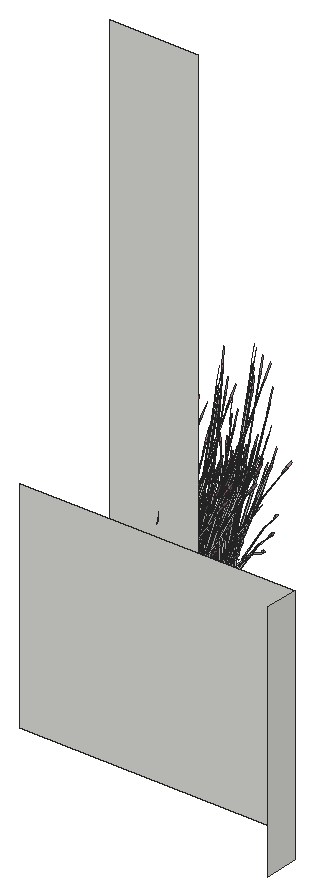
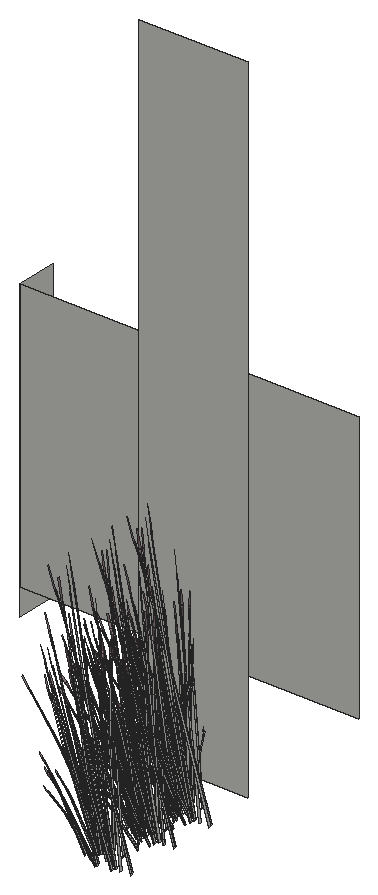
# SketchUp Ruby script. Lengths in inches.
U = 1.inch
M = Sketchup.active_model
def pt(a) = Geom::Point3d.new(a.map { |v| v * U })
def face(e, loops, mat)
  f = e.add_face(loops[0].map { |a| pt(a) })
  loops[1..].each { |l| e.add_face(l.map { |a| pt(a) }).erase! }
  f.material = f.back_material = mat if mat
  f
end
# faces: each face lists its corners as indices into pts; further lists are holes
def faces(e, pts, list, mat = nil) = list.each { |f| face(e, (f[0].is_a?(Array) ? f : [f]).map { |l| l.map { |i| pts[i] } }, mat) }
# xy, xz, yz: faces in a plane at the given z, y or x. An outline is a flat list of corners, or four numbers for a rectangle; further outlines are holes
def ring(l) = l.size == 4 ? [[l[0], l[1]], [l[2], l[1]], [l[2], l[3]], [l[0], l[3]]] : l.each_slice(2).to_a
def flat(e, list, mat, &to3) = list.each { |f| face(e, (f[0].is_a?(Array) ? f : [f]).map { |l| ring(l).map { |u, v| to3.(u, v) } }, mat) }
def xy(e, z, list, mat = nil) = flat(e, list, mat) { |x, y| [x, y, z] }
def xz(e, y, list, mat = nil) = flat(e, list, mat) { |x, z| [x, y, z] }
def yz(e, x, list, mat = nil) = flat(e, list, mat) { |y, z| [x, y, z] }
def lines(e, pts, list) = list.each { |a, b| e.add_line(pt(pts[a]), pt(pts[b])) }
# prism: a flat outline (further loops are holes) pulled along v
def prism(e, loops, v, mat = nil)
  f = face(e, loops, mat); d = Geom::Vector3d.new(v.map { |x| x * U })
  f.pushpull(f.normal.samedirection?(d) ? d.length : -d.length)
end
def box(e, o, s, mat = nil) = prism(e, [[o, [o[0] + s[0], o[1], o[2]], [o[0] + s[0], o[1] + s[1], o[2]], [o[0], o[1] + s[1], o[2]]]], [0, 0, s[2]], mat)
def at(x, y, z, deg = 0) = Geom::Transformation.translation(pt([x, y, z])) * Geom::Transformation.rotation(ORIGIN, Z_AXIS, deg.degrees)
def axes(o, x, y, z) = Geom::Transformation.new([*x, 0, *y, 0, *z, 0, *pt(o).to_a, 1])
def part(name) = M.definitions.add(name)
# library, detail: a bought-in or finely detailed component or shape, given as its bounding box
def library(name, o, s) = part(name).tap { |d| box(d.entities, o, s) }
def detail(e, o, s) = box(e.add_group.entities, o, s)
def put(e, d, t, mat = nil) = e.add_instance(d, t).tap { |i| i.material = mat if mat }
def group(e, t, mat = nil) = e.add_group.tap { |g| g.transformation = t; g.material = mat if mat }.entities
root = M.entities
M.materials.add("LightPink_Translucent").color = [144, 107, 117]
M.materials["LightPink_Translucent"].alpha = 0.75
c1 = part("blade")
p = [[2.15,0.21,22],[0,0.17,0],[0.09,0.45,0],[2.18,0.31,22],[2.29,0.31,22],[0.38,0.45,0],
  [2.48,0.24,33],[2.49,0.24,33],[2.48,0.22,33]]
faces(c1.entities,p,[[0,1,2,3],[4,5,2,3],[6,3,4,7],[8,0,3,6]])
c2 = part("seeds")
p = [[0.3,-0.1,1.38],[-0.01,-0.03,1.59],[-0.01,-0.03,0.03],[0.14,-0.07,-0.07],[0.29,-0.03,3],[0.15,0.01,3.11]]
faces(c2.entities,p,[[0,1,2,3],[1,0,4,5]],"LightPink_Translucent")
c3 = part("blade with seeds")
put(c3.entities,c1,at(0,0,0))
put(c3.entities,c2,axes([2.4,0.25,30.99],[1.5799,-0.05474,1.17369],[-0.12525,1.92788,0.29478],[-0.07173,-0.02425,1.56792]))
xz(root,9,[[351,0,426,60]])
xz(root,51,[[342,6,366,151.99]])
yz(root,426,[[0,-6,9,60]])
put(root,c3,axes([347.36,59.61,7.02],[0.73517,0.0304,0.0643],[-0.02016,0.45906,0.50621],[0.07693,-0.17585,0.77189]))
put(root,c3,axes([347.36,69.44,7.02],[0.73517,0.0304,0.0643],[-0.02016,0.45906,0.50621],[0.07693,-0.17585,0.77189]))
put(root,c3,axes([347.36,81.44,7.02],[0.73517,0.0304,0.0643],[-0.02016,0.45906,0.50621],[0.07693,-0.17585,0.77189]))
put(root,c3,axes([347.27,63.85,5.06],[-0.5037,-0.18761,1.1486],[0.6504,-0.19062,0.84392],[0.17543,0.16147,0.25299]))
put(root,c3,axes([347.27,73.68,5.06],[-0.5037,-0.18761,1.1486],[0.6504,-0.19062,0.84392],[0.17543,0.16147,0.25299]))
put(root,c3,axes([345.48,63.65,4.88],[0.01579,-0.21629,1.43002],[0.75442,-0.24159,-0.30754],[0.23289,0.25887,0.61141]))
put(root,c3,axes([345.48,73.48,4.88],[0.01579,-0.21629,1.43002],[0.75442,-0.24159,-0.30754],[0.23289,0.25887,0.61141]))
put(root,c3,axes([348.09,58.86,7.01],[-0.00864,-0.12985,1.74944],[-0.72937,-0.3753,-0.27667],[0.11277,-0.2275,0.14031]))
put(root,c3,axes([348.09,68.68,7.01],[-0.00864,-0.12985,1.74944],[-0.72937,-0.3753,-0.27667],[0.11277,-0.2275,0.14031]))
put(root,c3,axes([348.09,80.68,7.01],[-0.00864,-0.12985,1.74944],[-0.72937,-0.3753,-0.27667],[0.11277,-0.2275,0.14031]))
put(root,c3,axes([344.57,60.59,4.35],[0.60257,-0.49041,-0.62353],[0.74854,0.44469,-0.16365],[0.24146,-0.12234,1.37633]))
put(root,c3,axes([344.57,70.41,4.35],[0.60257,-0.49041,-0.62353],[0.74854,0.44469,-0.16365],[0.24146,-0.12234,1.37633]))
put(root,c3,axes([344.57,82.41,4.35],[0.60257,-0.49041,-0.62353],[0.74854,0.44469,-0.16365],[0.24146,-0.12234,1.37633]))
put(root,c3,axes([347.12,59.57,7.03],[0.63704,0.44518,0.48003],[-0.67652,0.38394,0.3958],[0.11751,-0.20886,0.9933]))
put(root,c3,axes([347.12,69.4,7.03],[0.63704,0.44518,0.48003],[-0.67652,0.38394,0.3958],[0.11751,-0.20886,0.9933]))
put(root,c3,axes([347.12,81.4,7.03],[0.63704,0.44518,0.48003],[-0.67652,0.38394,0.3958],[0.11751,-0.20886,0.9933]))
put(root,c3,axes([347.22,60.15,4.32],[0.21015,0.56852,-0.30978],[-0.83462,0.16144,0.30978],[0.16826,0.06556,1.38974]))
put(root,c3,axes([347.22,69.98,4.32],[0.21015,0.56852,-0.30978],[-0.83462,0.16144,0.30978],[0.16826,0.06556,1.38974]))
put(root,c3,axes([347.22,81.98,4.32],[0.21015,0.56852,-0.30978],[-0.83462,0.16144,0.30978],[0.16826,0.06556,1.38974]))
put(root,c3,axes([348.79,62.01,4.67],[1.11865,0,0],[0,0.72922,-0.51607],[0,0.16609,1.63711]))
put(root,c3,axes([348.79,71.83,4.67],[1.11865,0,0],[0,0.72922,-0.51607],[0,0.16609,1.63711]))
put(root,c3,axes([345.17,61.06,4.96],[0.90324,-0.43318,-0.29095],[0.60064,0.61207,-0.50002],[0.22285,0.06216,1.59708]))
put(root,c3,axes([345.17,70.89,4.96],[0.90324,-0.43318,-0.29095],[0.60064,0.61207,-0.50002],[0.22285,0.06216,1.59708]))
put(root,c3,axes([345.17,82.89,4.96],[0.90324,-0.43318,-0.29095],[0.60064,0.61207,-0.50002],[0.22285,0.06216,1.59708]))
put(root,c3,axes([347.35,64.71,4.96],[-0.57368,-0.02046,1.0506],[0.37886,-0.43461,0.58006],[0.22663,0.15441,0.8241]))
put(root,c3,axes([347.35,74.53,4.96],[-0.57368,-0.02046,1.0506],[0.37886,-0.43461,0.58006],[0.22663,0.15441,0.8241]))
put(root,c3,axes([347.86,60.99,7.34],[-0.77872,0.09325,0.35414],[-0.20563,-0.53305,-0.4572],[0.22316,-0.14318,0.87481]))
put(root,c3,axes([347.86,70.8125,7.34],[-0.77872,0.09325,0.35414],[-0.20563,-0.53305,-0.4572],[0.22316,-0.14318,0.87481]))
put(root,c3,axes([347.86,82.8125,7.34],[-0.77872,0.09325,0.35414],[-0.20563,-0.53305,-0.4572],[0.22316,-0.14318,0.87481]))
put(root,c3,axes([345.62,59.49,6.17],[-0.16657,0.22426,1.71376],[-0.69879,-0.4641,0.13857],[0.31524,-0.28926,0.73262]))
put(root,c3,axes([345.62,69.32,6.17],[-0.16657,0.22426,1.71376],[-0.69879,-0.4641,0.13857],[0.31524,-0.28926,0.73262]))
put(root,c3,axes([345.62,81.32,6.17],[-0.16657,0.22426,1.71376],[-0.69879,-0.4641,0.13857],[0.31524,-0.28926,0.73262]))
put(root,c3,axes([345.5,64.39,7.33],[0.53309,-0.55848,-0.1216],[0.77201,0.32175,-0.67495],[0.26836,0.15779,1.02557]))
put(root,c3,axes([345.5,74.22,7.33],[0.53309,-0.55848,-0.1216],[0.77201,0.32175,-0.67495],[0.26836,0.15779,1.02557]))
put(root,c3,axes([342.89,60.67,3.89],[-0.88056,0.26122,1.28929],[-0.28027,-0.74951,0.50096],[0.54072,0.01247,1.46642]))
put(root,c3,axes([342.89,70.5,3.89],[-0.88056,0.26122,1.28929],[-0.28027,-0.74951,0.50096],[0.54072,0.01247,1.46642]))
put(root,c3,axes([342.89,82.5,3.89],[-0.88056,0.26122,1.28929],[-0.28027,-0.74951,0.50096],[0.54072,0.01247,1.46642]))
put(root,c3,axes([348.26,61.03,7.33],[-0.82753,-0.35977,-0.1216],[0.47675,-0.52101,-0.67495],[0.2338,-0.18111,1.02557]))
put(root,c3,axes([348.26,70.86,7.33],[-0.82753,-0.35977,-0.1216],[0.47675,-0.52101,-0.67495],[0.2338,-0.18111,1.02557]))
put(root,c3,axes([348.26,82.86,7.33],[-0.82753,-0.35977,-0.1216],[0.47675,-0.52101,-0.67495],[0.2338,-0.18111,1.02557]))
put(root,c3,axes([346.13,64.11,6.97],[0.88277,-0.1551,-0.51099],[0.15442,0.58737,-0.3958],[0.23711,0.16832,0.97773]))
put(root,c3,axes([346.13,73.9375,6.97],[0.88277,-0.1551,-0.51099],[0.15442,0.58737,-0.3958],[0.23711,0.16832,0.97773]))
put(root,c3,axes([346.94,59.52,4.67],[0.55932,-0.6538,0],[0.93577,0.36461,-0.51607],[0.21313,0.08304,1.63711]))
put(root,c3,axes([346.94,69.34,4.67],[0.55932,-0.6538,0],[0.93577,0.36461,-0.51607],[0.21313,0.08304,1.63711]))
put(root,c3,axes([346.94,81.34,4.67],[0.55932,-0.6538,0],[0.93577,0.36461,-0.51607],[0.21313,0.08304,1.63711]))
put(root,c3,axes([347.88,59.23,3.79],[-0.1339,-0.0514,1.76342],[-0.34394,-0.57425,-0.26939],[0.23202,-0.15583,0.30037]))
put(root,c3,axes([347.88,69.06,3.79],[-0.1339,-0.0514,1.76342],[-0.34394,-0.57425,-0.26939],[0.23202,-0.15583,0.30037]))
put(root,c3,axes([347.88,81.06,3.79],[-0.1339,-0.0514,1.76342],[-0.34394,-0.57425,-0.26939],[0.23202,-0.15583,0.30037]))
put(root,c3,axes([347.14,63.41,7.34],[-0.50902,-0.40851,0.35414],[0.58122,-0.38671,-0.4572],[0.29531,0.05884,0.87481]))
put(root,c3,axes([347.14,73.23,7.34],[-0.50902,-0.40851,0.35414],[0.58122,-0.38671,-0.4572],[0.29531,0.05884,0.87481]))
put(root,c3,axes([347.45,59.91,4.3125],[0.83726,0.32623,-0.49651],[-0.50045,0.58498,0],[0.19069,0.0743,1.57504]))
put(root,c3,axes([347.45,69.74,4.3125],[0.83726,0.32623,-0.49651],[-0.50045,0.58498,0],[0.19069,0.0743,1.57504]))
put(root,c3,axes([347.45,81.74,4.3125],[0.83726,0.32623,-0.49651],[-0.50045,0.58498,0],[0.19069,0.0743,1.57504]))
put(root,c3,axes([347.61,63.78,7.02],[-0.04505,0.49615,0.0643],[-0.68022,-0.0136,0.50621],[0.26056,0.05192,0.77189]))
put(root,c3,axes([347.61,73.6,7.02],[-0.04505,0.49615,0.0643],[-0.68022,-0.0136,0.50621],[0.26056,0.05192,0.77189]))
put(root,c3,axes([347.41,64.55,3.79],[0.06518,-0.0942,1.76342],[0.82057,-0.27742,-0.26939],[0.24877,0.14358,0.30037]))
put(root,c3,axes([347.41,74.375,3.79],[0.06518,-0.0942,1.76342],[0.82057,-0.27742,-0.26939],[0.24877,0.14358,0.30037]))
put(root,c3,axes([347.67,63.62,7.03],[-0.65964,0.42992,0.48003],[-0.5689,-0.45657,0.3958],[0.30948,0.0793,0.9933]))
put(root,c3,axes([347.67,73.45,7.03],[-0.65964,0.42992,0.48003],[-0.5689,-0.45657,0.3958],[0.30948,0.0793,0.9933]))
put(root,c3,axes([347.85,60.61,6.97],[-0.22982,-0.59576,-0.51099],[0.87033,-0.10422,-0.3958],[0.24941,-0.16002,0.97773]))
put(root,c3,axes([347.85,70.44,6.97],[-0.22982,-0.59576,-0.51099],[0.87033,-0.10422,-0.3958],[0.24941,-0.16002,0.97773]))
put(root,c3,axes([347.85,82.44,6.97],[-0.22982,-0.59576,-0.51099],[0.87033,-0.10422,-0.3958],[0.24941,-0.16002,0.97773]))
put(root,c3,axes([349.38,63.68,6.22],[-0.17122,-0.54847,-0.03492],[0.80929,-0.12609,-0.15832],[0.169,0.03477,0.52218]))
put(root,c3,axes([349.38,73.51,6.22],[-0.17122,-0.54847,-0.03492],[0.80929,-0.12609,-0.15832],[0.169,0.03477,0.52218]))
put(root,c3,axes([347.98,62.26,7.34],[-0.74348,-0.18202,0.35414],[0.21685,-0.53102,-0.4572],[0.29933,-0.04869,0.87481]))
put(root,c3,axes([347.98,72.09,7.34],[-0.74348,-0.18202,0.35414],[0.21685,-0.53102,-0.4572],[0.29933,-0.04869,0.87481]))
put(root,c3,axes([347.98,84.09,7.34],[-0.74348,-0.18202,0.35414],[0.21685,-0.53102,-0.4572],[0.29933,-0.04869,0.87481]))
put(root,c3,axes([346.23,61.16,4.35],[0.9306,0.10697,-0.62353],[-0.19638,0.65984,-0.16365],[0.27771,0.07995,1.37633]))
put(root,c3,axes([346.23,70.98,4.35],[0.9306,0.10697,-0.62353],[-0.19638,0.65984,-0.16365],[0.27771,0.07995,1.37633]))
put(root,c3,axes([346.23,82.98,4.35],[0.9306,0.10697,-0.62353],[-0.19638,0.65984,-0.16365],[0.27771,0.07995,1.37633]))
put(root,c3,axes([350.19,61.55,4.55],[-0.55463,-0.41721,-0.06488],[0.60744,-0.38228,-0.29416],[0.17212,-0.02691,0.97024]))
put(root,c3,axes([350.19,71.375,4.55],[-0.55463,-0.41721,-0.06488],[0.60744,-0.38228,-0.29416],[0.17212,-0.02691,0.97024]))
put(root,c3,axes([350.19,83.375,4.55],[-0.55463,-0.41721,-0.06488],[0.60744,-0.38228,-0.29416],[0.17212,-0.02691,0.97024]))
put(root,c3,axes([348.92,59.42,5.06],[-0.29798,0.33213,1.1486],[-0.25612,-0.44624,0.84392],[0.24611,-0.11182,0.25299]))
put(root,c3,axes([348.92,69.25,5.06],[-0.29798,0.33213,1.1486],[-0.25612,-0.44624,0.84392],[0.24611,-0.11182,0.25299]))
put(root,c3,axes([348.92,81.25,5.06],[-0.29798,0.33213,1.1486],[-0.25612,-0.44624,0.84392],[0.24611,-0.11182,0.25299]))
put(root,c3,axes([348.5625,60.9,7.02],[0.61415,0.2744,0.0643],[-0.35756,0.39076,0.50621],[0.1969,-0.12633,0.77189]))
put(root,c3,axes([348.5625,70.73,7.02],[0.61415,0.2744,0.0643],[-0.35756,0.39076,0.50621],[0.1969,-0.12633,0.77189]))
put(root,c3,axes([348.5625,82.73,7.02],[0.61415,0.2744,0.0643],[-0.35756,0.39076,0.50621],[0.1969,-0.12633,0.77189]))
put(root,c3,axes([348.39,60.79,7.03],[0.22187,0.60049,0.48003],[-0.87033,0.10422,0.3958],[0.25651,-0.14123,0.9933]))
put(root,c3,axes([348.39,70.61,7.03],[0.22187,0.60049,0.48003],[-0.87033,0.10422,0.3958],[0.25651,-0.14123,0.9933]))
put(root,c3,axes([348.39,82.61,7.03],[0.22187,0.60049,0.48003],[-0.87033,0.10422,0.3958],[0.25651,-0.14123,0.9933]))
put(root,c3,axes([346.04,62.57,6.17],[-0.3323,-0.11241,1.71376],[0.68769,-0.4716,0.13857],[0.42861,0.21275,0.73262]))
put(root,c3,axes([346.04,72.4,6.17],[-0.3323,-0.11241,1.71376],[0.68769,-0.4716,0.13857],[0.42861,0.21275,0.73262]))
put(root,c3,axes([350.3,60.88,7],[-0.11685,-0.00496,1.77383],[-0.48522,-0.53096,-0.16761],[0.19486,-0.17458,0.31391]))
put(root,c3,axes([350.3,70.71,7],[-0.11685,-0.00496,1.77383],[-0.48522,-0.53096,-0.16761],[0.19486,-0.17458,0.31391]))
put(root,c3,axes([350.3,82.71,7],[-0.11685,-0.00496,1.77383],[-0.48522,-0.53096,-0.16761],[0.19486,-0.17458,0.31391]))
put(root,c3,axes([348.49,60.67,6.82],[0.77872,-0.09325,-0.35414],[0.20563,0.53305,0.4572],[0.22316,-0.14318,0.87481]))
put(root,c3,axes([348.49,70.5,6.82],[0.77872,-0.09325,-0.35414],[0.20563,0.53305,0.4572],[0.22316,-0.14318,0.87481]))
put(root,c3,axes([348.49,82.5,6.82],[0.77872,-0.09325,-0.35414],[0.20563,0.53305,0.4572],[0.22316,-0.14318,0.87481]))
put(root,c3,axes([347.875,60.85,7.27],[0.4673,-0.51481,-0.71045],[0.81887,0.36587,0.08574],[0.27902,-0.18652,1.00501]))
put(root,c3,axes([347.875,70.68,7.27],[0.4673,-0.51481,-0.71045],[0.81887,0.36587,0.08574],[0.27902,-0.18652,1.00501]))
put(root,c3,axes([347.875,82.68,7.27],[0.4673,-0.51481,-0.71045],[0.81887,0.36587,0.08574],[0.27902,-0.18652,1.00501]))
put(root,c3,axes([348.66,62.43,7.02],[0.32857,0.44488,0.0643],[-0.59916,0.21775,0.50621],[0.26412,-0.04296,0.77189]))
put(root,c3,axes([348.66,72.25,7.02],[0.32857,0.44488,0.0643],[-0.59916,0.21775,0.50621],[0.26412,-0.04296,0.77189]))
put(root,c3,axes([348.66,84.25,7.02],[0.32857,0.44488,0.0643],[-0.59916,0.21775,0.50621],[0.26412,-0.04296,0.77189]))
put(root,c3,axes([347.87,63.62,6.82],[0.50902,0.40851,-0.35414],[-0.58122,0.38671,0.4572],[0.29531,0.05884,0.87481]))
put(root,c3,axes([347.87,73.45,6.82],[0.50902,0.40851,-0.35414],[-0.58122,0.38671,0.4572],[0.29531,0.05884,0.87481]))
put(root,c3,axes([347.28,63.67,7.33],[0.0479,-0.66354,-0.1216],[0.90696,0.01814,-0.67495],[0.3493,0.04609,1.02557]))
put(root,c3,axes([347.28,73.49,7.33],[0.0479,-0.66354,-0.1216],[0.90696,0.01814,-0.67495],[0.3493,0.04609,1.02557]))
put(root,c3,axes([348.29,62.4375,7.33],[-0.45012,-0.59081,-0.1216],[0.79888,-0.29033,-0.67495],[0.33665,-0.07795,1.02557]))
put(root,c3,axes([348.29,72.27,7.33],[-0.45012,-0.59081,-0.1216],[0.79888,-0.29033,-0.67495],[0.33665,-0.07795,1.02557]))
put(root,c3,axes([348.29,84.27,7.33],[-0.45012,-0.59081,-0.1216],[0.79888,-0.29033,-0.67495],[0.33665,-0.07795,1.02557]))
put(root,c3,axes([348.59,62.27,7.03],[-0.25275,0.59491,0.48003],[-0.83094,-0.20343,0.3958],[0.32677,-0.03575,0.9933]))
put(root,c3,axes([348.59,72.09,7.03],[-0.25275,0.59491,0.48003],[-0.83094,-0.20343,0.3958],[0.32677,-0.03575,0.9933]))
put(root,c3,axes([348.59,84.09,7.03],[-0.25275,0.59491,0.48003],[-0.83094,-0.20343,0.3958],[0.32677,-0.03575,0.9933]))
put(root,c3,axes([348.07,63.27,7.01],[0.19191,-0.01103,1.74944],[0.52639,-0.5069,-0.27667],[0.34136,0.06691,0.14031]))
put(root,c3,axes([348.07,73.1,7.01],[0.19191,-0.01103,1.74944],[0.52639,-0.5069,-0.27667],[0.34136,0.06691,0.14031]))
put(root,c3,axes([348.26,61.93,6.97],[0.24236,-0.59349,-0.51099],[0.83094,0.20343,-0.3958],[0.33455,-0.05442,0.97773]))
put(root,c3,axes([348.26,71.76,6.97],[0.24236,-0.59349,-0.51099],[0.83094,0.20343,-0.3958],[0.33455,-0.05442,0.97773]))
put(root,c3,axes([348.26,83.76,6.97],[0.24236,-0.59349,-0.51099],[0.83094,0.20343,-0.3958],[0.33455,-0.05442,0.97773]))
put(root,c3,axes([350.34,62.31,5.06],[-0.55274,0.10771,1.1486],[0.26018,-0.44517,0.84392],[0.29323,0.03046,0.25299]))
put(root,c3,axes([350.34,72.14,5.06],[-0.55274,0.10771,1.1486],[0.26018,-0.44517,0.84392],[0.29323,0.03046,0.25299]))
put(root,c3,axes([350.34,84.14,5.06],[-0.55274,0.10771,1.1486],[0.26018,-0.44517,0.84392],[0.29323,0.03046,0.25299]))
put(root,c3,axes([348.55,60.375,4.88],[-0.31959,-0.01933,1.43002],[-0.32741,-0.51843,-0.30754],[0.39262,-0.14666,0.61141]))
put(root,c3,axes([348.55,70.2,4.88],[-0.31959,-0.01933,1.43002],[-0.32741,-0.51843,-0.30754],[0.39262,-0.14666,0.61141]))
put(root,c3,axes([348.55,82.2,4.88],[-0.31959,-0.01933,1.43002],[-0.32741,-0.51843,-0.30754],[0.39262,-0.14666,0.61141]))
put(root,c3,axes([348.76,62.2,6.82],[0.74348,0.18202,-0.35414],[-0.21685,0.53102,0.4572],[0.29933,-0.04869,0.87481]))
put(root,c3,axes([348.76,72.03,6.82],[0.74348,0.18202,-0.35414],[-0.21685,0.53102,0.4572],[0.29933,-0.04869,0.87481]))
put(root,c3,axes([348.76,84.03,6.82],[0.74348,0.18202,-0.35414],[-0.21685,0.53102,0.4572],[0.29933,-0.04869,0.87481]))
put(root,c3,axes([347.33,63.35,7.27],[0.89428,0.01571,-0.71045],[-0.06006,0.66153,0.08574],[0.37886,0.06981,1.00501]))
put(root,c3,axes([347.33,73.17,7.27],[0.89428,0.01571,-0.71045],[-0.06006,0.66153,0.08574],[0.37886,0.06981,1.00501]))
put(root,c3,axes([349.14,62.1,4.28],[-0.57619,0.0783,1.41583],[-0.09171,-0.62326,0.08104],[0.40356,-0.09434,0.80566]))
put(root,c3,axes([349.14,71.93,4.28],[-0.57619,0.0783,1.41583],[-0.09171,-0.62326,0.08104],[0.40356,-0.09434,0.80566]))
put(root,c3,axes([349.14,83.93,4.28],[-0.57619,0.0783,1.41583],[-0.09171,-0.62326,0.08104],[0.40356,-0.09434,0.80566]))
put(root,c3,axes([349.77,61.69,3.79],[-0.04675,-0.09906,1.76342],[0.32428,-0.57943,-0.26939],[0.32711,-0.00833,0.30037]))
put(root,c3,axes([349.77,71.52,3.79],[-0.04675,-0.09906,1.76342],[0.32428,-0.57943,-0.26939],[0.32711,-0.00833,0.30037]))
put(root,c3,axes([349.77,83.52,3.79],[-0.04675,-0.09906,1.76342],[0.32428,-0.57943,-0.26939],[0.32711,-0.00833,0.30037]))
put(root,c3,axes([350.09,64.19,7],[-0.08089,-0.05712,1.77383],[0.17695,-0.61228,-0.16761],[0.31864,-0.03912,0.31391]))
put(root,c3,axes([350.09,74.02,7],[-0.08089,-0.05712,1.77383],[0.17695,-0.61228,-0.16761],[0.31864,-0.03912,0.31391]))
put(root,c3,axes([350.09,86.02,7],[-0.08089,-0.05712,1.77383],[0.17695,-0.61228,-0.16761],[0.31864,-0.03912,0.31391]))
put(root,c3,axes([346.74,61.55,6.17],[-0.37107,0.01478,1.71376],[0.24616,-0.64047,0.13857],[0.5288,0.03961,0.73262]))
put(root,c3,axes([346.74,71.37,6.17],[-0.37107,0.01478,1.71376],[0.24616,-0.64047,0.13857],[0.5288,0.03961,0.73262]))
put(root,c3,axes([346.74,83.37,6.17],[-0.37107,0.01478,1.71376],[0.24616,-0.64047,0.13857],[0.5288,0.03961,0.73262]))
put(root,c3,axes([348.1,62.15,7.27],[0.78611,-0.28816,-0.71045],[0.4381,0.59317,0.08574],[0.37982,-0.06738,1.00501]))
put(root,c3,axes([348.1,71.97,7.27],[0.78611,-0.28816,-0.71045],[0.4381,0.59317,0.08574],[0.37982,-0.06738,1.00501]))
put(root,c3,axes([348.1,83.97,7.27],[0.78611,-0.28816,-0.71045],[0.4381,0.59317,0.08574],[0.37982,-0.06738,1.00501]))
put(root,c3,axes([350.74,61.51,7.01],[0.12414,-0.09938,1.74944],[-0.15889,-0.60963,-0.27667],[0.31148,-0.11559,0.14031]))
put(root,c3,axes([350.74,71.34,7.01],[0.12414,-0.09938,1.74944],[-0.15889,-0.60963,-0.27667],[0.31148,-0.11559,0.14031]))
put(root,c3,axes([350.74,83.34,7.01],[0.12414,-0.09938,1.74944],[-0.15889,-0.60963,-0.27667],[0.31148,-0.11559,0.14031]))
put(root,c3,axes([349.31,63.02,4.88],[-0.21545,-0.16047,1.43002],[0.28033,-0.53085,-0.30754],[0.43591,0.07191,0.61141]))
put(root,c3,axes([349.31,72.85,4.88],[-0.21545,-0.16047,1.43002],[0.28033,-0.53085,-0.30754],[0.43591,0.07191,0.61141]))
